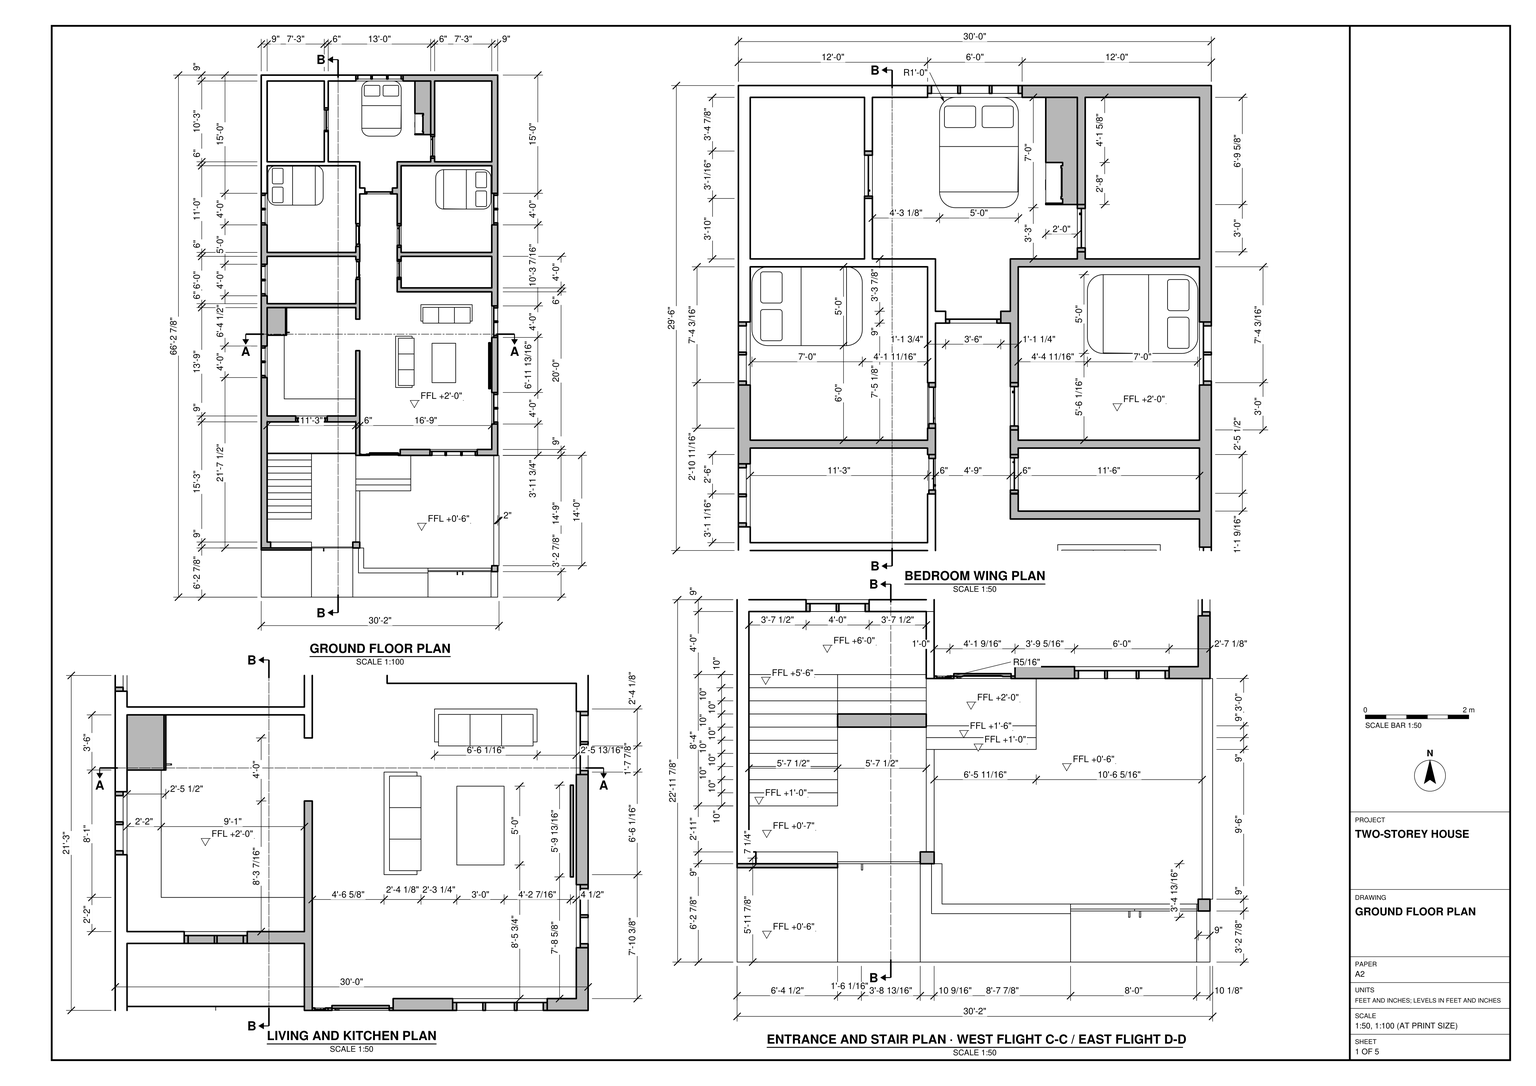
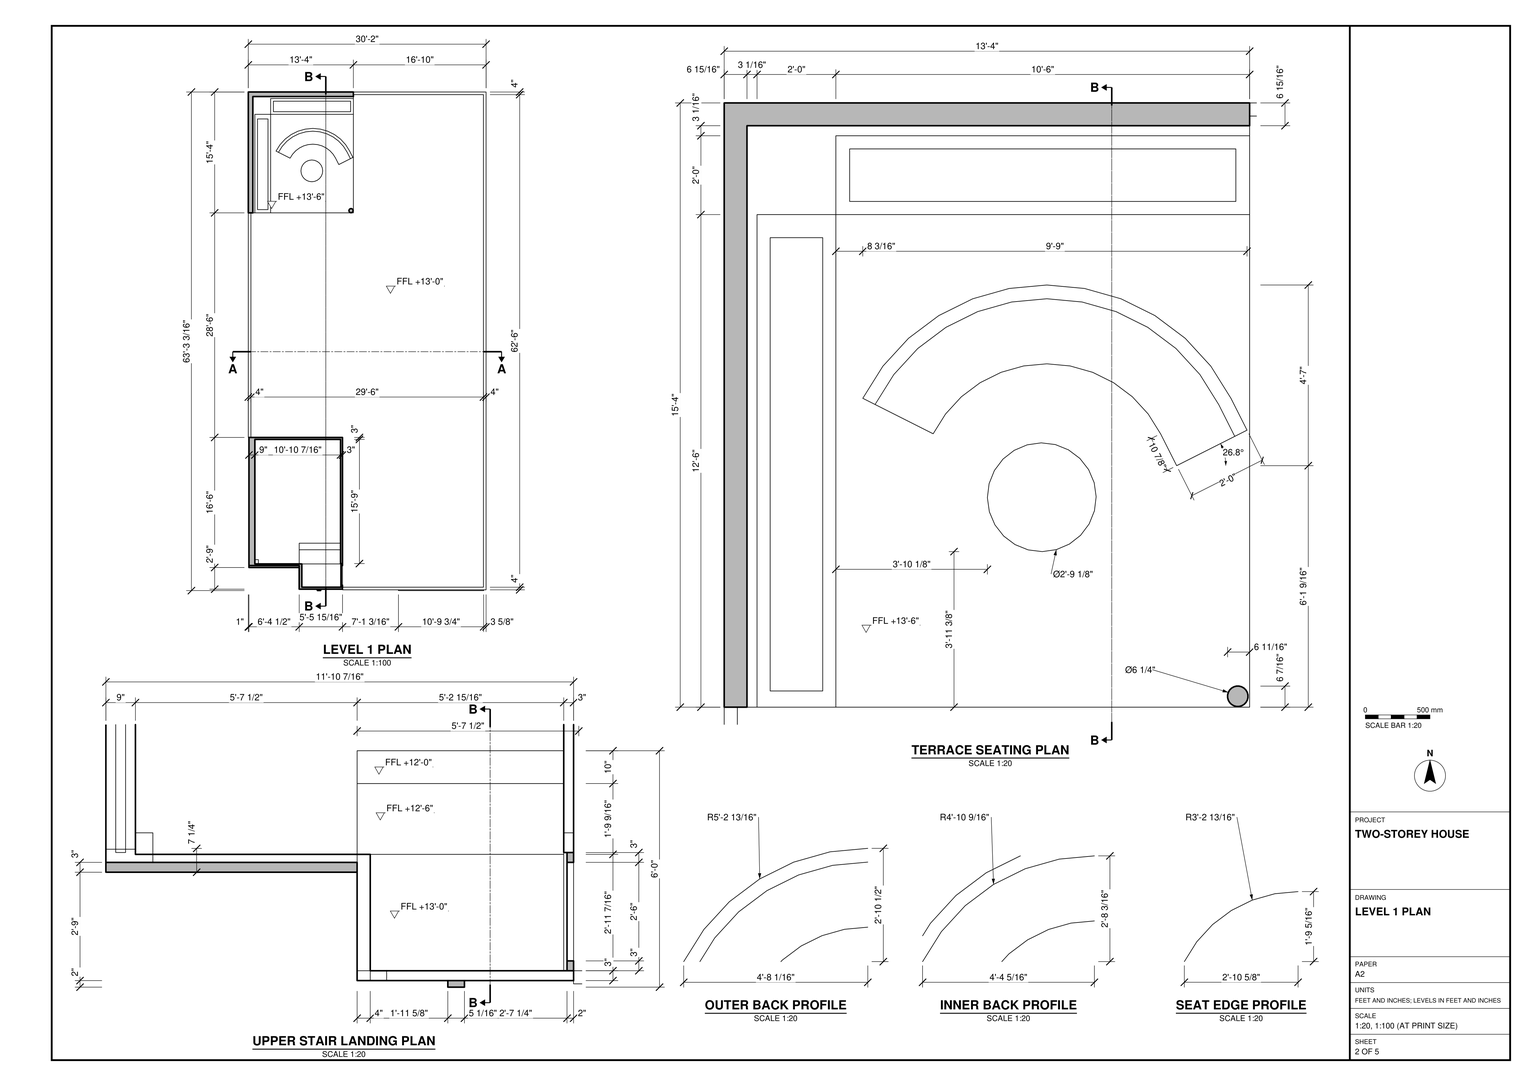
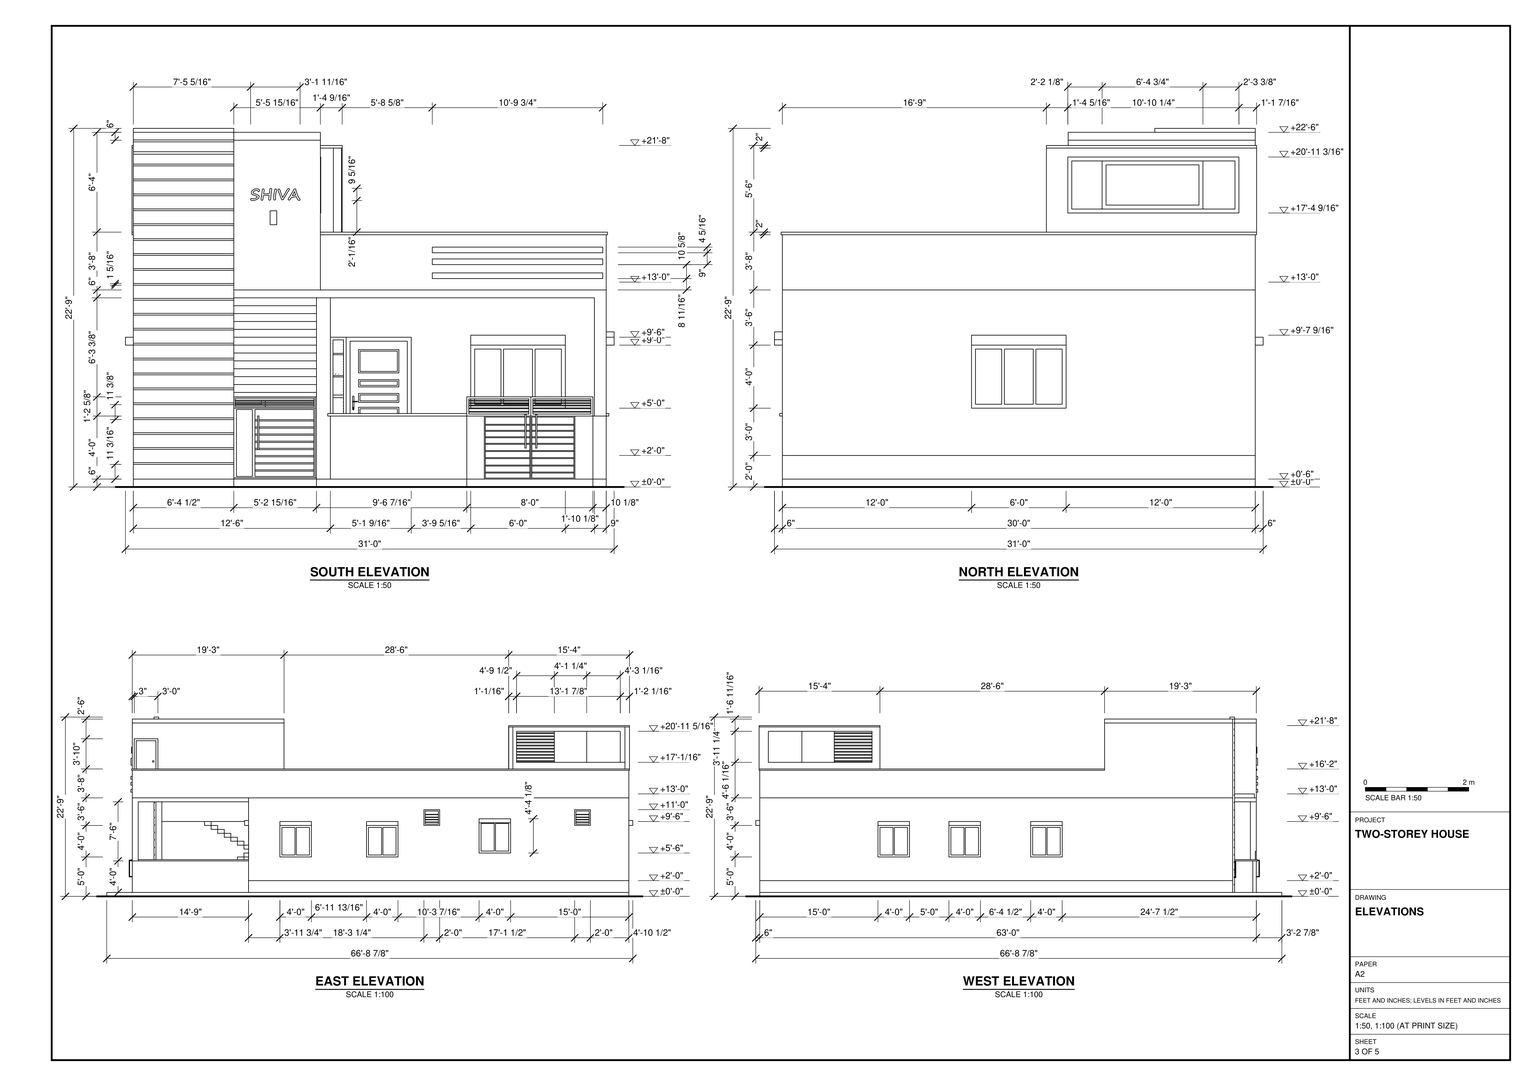
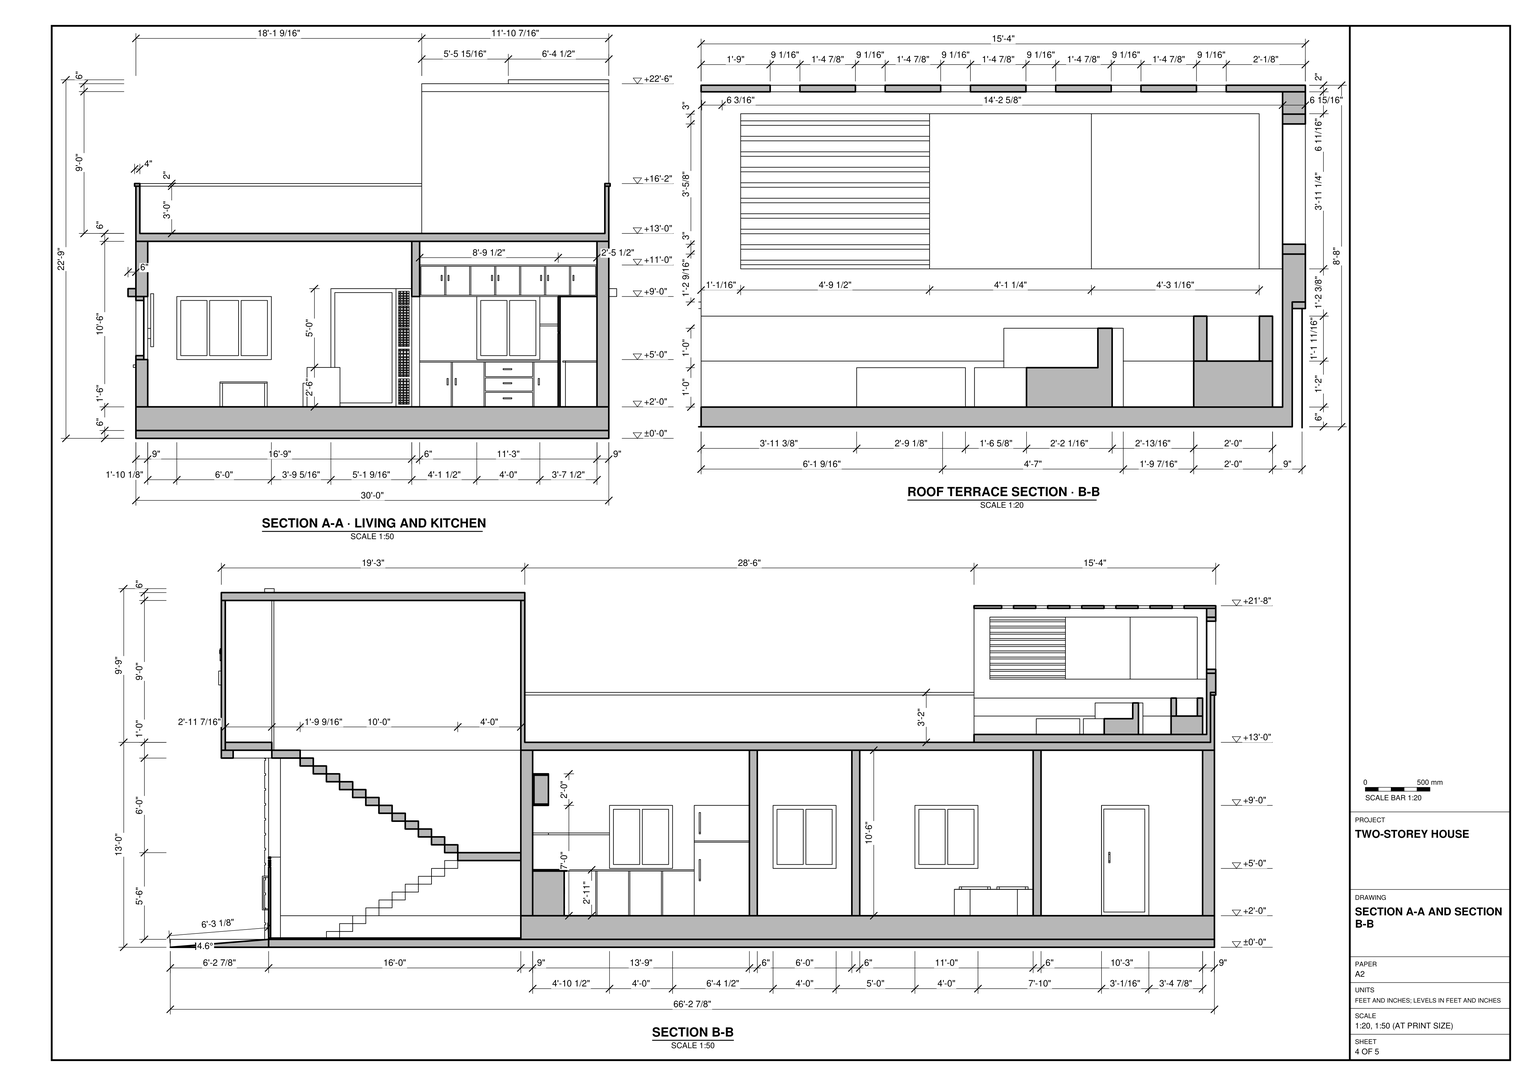
Build the house in SketchUp from task_files/diagram_01.pdf. Work in feet and inches. Set the overall width to 31'-0", the front-to-back length to 66'-8 7/8" and the height to 22'-9". Use ±0'-0" as the ground-floor datum and +13'-0" as the upper storey level. Distinguish these levels from the raised floor surfaces shown on the plans.

Start at the south entrance. Model the front gates, porch, entry steps and return stair, including its intermediate and upper landings. Place the living area and kitchen behind the porch, with a passage leading to the rear bedroom wing. Follow the drawn wall thicknesses, including the 9" exterior walls and 6" partitions where indicated. Form the door, window and vent openings to match the plans and elevations. Include the kitchen joinery, bedroom storage, beds, living room seating and rectangular table in their drawn positions.

Model the floor and roof slabs, terrace parapets and raised stair enclosure. At the opposite end of the terrace, reproduce the raised seating area with its curved seat and round table. Use the elevations to set out the horizontal bands on the entrance front and the openings along both sides. Decor and loose items may be any suitable library components.

Keep shell elements such as walls, slabs and roof, and each furniture or joinery piece, in separate groups or components. Use components for repeated parts. Save one SketchUp model as output_files/two_storey_house_with_a_furnished_roof_terrace.skp.

# SketchUp Ruby script. Lengths in inches.
U = 1.inch
M = Sketchup.active_model
def pt(a) = Geom::Point3d.new(a.map { |v| v * U })
def face(e, loops, mat)
  f = e.add_face(loops[0].map { |a| pt(a) })
  loops[1..].each { |l| e.add_face(l.map { |a| pt(a) }).erase! }
  f.material = f.back_material = mat if mat
  f
end
# faces: each face lists its corners as indices into pts; further lists are holes
def faces(e, pts, list, mat = nil) = list.each { |f| face(e, (f[0].is_a?(Array) ? f : [f]).map { |l| l.map { |i| pts[i] } }, mat) }
# xy, xz, yz: faces in a plane at the given z, y or x. An outline is a flat list of corners, or four numbers for a rectangle; further outlines are holes
def ring(l) = l.size == 4 ? [[l[0], l[1]], [l[2], l[1]], [l[2], l[3]], [l[0], l[3]]] : l.each_slice(2).to_a
def flat(e, list, mat, &to3) = list.each { |f| face(e, (f[0].is_a?(Array) ? f : [f]).map { |l| ring(l).map { |u, v| to3.(u, v) } }, mat) }
def xy(e, z, list, mat = nil) = flat(e, list, mat) { |x, y| [x, y, z] }
def xz(e, y, list, mat = nil) = flat(e, list, mat) { |x, z| [x, y, z] }
def yz(e, x, list, mat = nil) = flat(e, list, mat) { |y, z| [x, y, z] }
def lines(e, pts, list) = list.each { |a, b| e.add_line(pt(pts[a]), pt(pts[b])) }
# prism: a flat outline (further loops are holes) pulled along v
def prism(e, loops, v, mat = nil)
  f = face(e, loops, mat); d = Geom::Vector3d.new(v.map { |x| x * U })
  f.pushpull(f.normal.samedirection?(d) ? d.length : -d.length)
end
def box(e, o, s, mat = nil) = prism(e, [[o, [o[0] + s[0], o[1], o[2]], [o[0] + s[0], o[1] + s[1], o[2]], [o[0], o[1] + s[1], o[2]]]], [0, 0, s[2]], mat)
def at(x, y, z, deg = 0) = Geom::Transformation.translation(pt([x, y, z])) * Geom::Transformation.rotation(ORIGIN, Z_AXIS, deg.degrees)
def axes(o, x, y, z) = Geom::Transformation.new([*x, 0, *y, 0, *z, 0, *pt(o).to_a, 1])
def part(name) = M.definitions.add(name)
# library, detail: a bought-in or finely detailed component or shape, given as its bounding box
def library(name, o, s) = part(name).tap { |d| box(d.entities, o, s) }
def detail(e, o, s) = box(e.add_group.entities, o, s)
def put(e, d, t, mat = nil) = e.add_instance(d, t).tap { |i| i.material = mat if mat }
def group(e, t, mat = nil) = e.add_group.tap { |g| g.transformation = t; g.material = mat if mat }.entities
root = M.entities
M.materials.add("A01_Blush_Petal").color = [255, 204, 204]
M.materials.add("B01_Ivory_Dust").color = [255, 217, 206]
M.materials.add("Carpet_1_1K").color = [242, 174, 12]
M.materials.add("G01_Mint_Mist").color = [204, 255, 204]
M.materials.add("Glass_Basic_01").color = [161, 173, 186]
M.materials["Glass_Basic_01"].alpha = 0.25
M.materials.add("Glass_Mirror_01").color = [185, 185, 185]
M.materials.add("M00_Soft_Cloud").color = [255, 255, 255]
M.materials.add("M02_Ash_Whisper").color = [196, 196, 196]
M.materials.add("M04_Stone_Frost").color = [142, 142, 142]
M.materials.add("M05_Graphite_Haze").color = [114, 114, 114]
M.materials.add("M06_Steel_Smoke").color = [86, 86, 86]
M.materials.add("M07_Charcoal_Gleam").color = [58, 58, 58]
M.materials.add("M08_Obsidian_Black").color = [30, 30, 30]
M.materials.add("M09_Shadow_Night").color = [0, 0, 0]
M.materials.add("Marble_01_1K").color = [230, 221, 211]
M.materials.add("Marble_03_1K").color = [175, 182, 201]
M.materials.add("Marble_06_1K").color = [165, 150, 147]
M.materials.add("Marble_20_1K").color = [172, 173, 182]
M.materials.add("Metal_06_1K").color = [220, 236, 231]
M.materials.add("Metal_10_1K").color = [196, 175, 123]
M.materials.add("Plaster_02_1K").color = [157, 140, 119]
M.materials.add("Plaster_04_1K").color = [106, 98, 87]
M.materials.add("Plywood_01_1K").color = [125, 96, 64]
M.materials.add("Soil_04_1K").color = [152, 146, 88]
M.materials.add("Wood_Floor_01_1K").color = [146, 111, 76]
M.materials.add("Wood_Floor_12_1K").color = [92, 75, 65]
M.materials.add("Wood_Veneer_15_1K").color = [103, 69, 45]
c1 = library("SHIVA",[0.42,0,0],[37.67,9.31,1])
c2 = part("Group\#4")
xy(c2.entities,0,[[0,-6,72,0]],"M09_Shadow_Night")
xy(c2.entities,3,[[3,-6,23,0],[25,-6,47,0],[49,-6,69,0]],"M09_Shadow_Night")
xy(c2.entities,45,[[3,-6,23,0],[25,-6,47,0],[49,-6,69,0]],"M09_Shadow_Night")
xy(c2.entities,48,[[0,-6,72,0]],"M09_Shadow_Night")
xz(c2.entities,-6,[[[0,0,72,48],[25,3,47,45],[3,3,23,45],[49,3,69,45]]],"M09_Shadow_Night")
xz(c2.entities,0,[[3,3,23,45],[25,3,47,45],[49,3,69,45]],"Glass_Basic_01")
xz(c2.entities,0,[[[0,0,72,48],[25,3,47,45],[3,3,23,45],[49,3,69,45]]],"M09_Shadow_Night")
yz(c2.entities,0,[[-6,0,0,48]],"M09_Shadow_Night")
yz(c2.entities,3,[[-6,3,0,45]],"M09_Shadow_Night")
yz(c2.entities,23,[[-6,3,0,45]],"M09_Shadow_Night")
yz(c2.entities,25,[[-6,3,0,45]],"M09_Shadow_Night")
yz(c2.entities,47,[[-6,3,0,45]],"M09_Shadow_Night")
yz(c2.entities,49,[[-6,3,0,45]],"M09_Shadow_Night")
yz(c2.entities,69,[[-6,3,0,45]],"M09_Shadow_Night")
yz(c2.entities,72,[[-6,0,0,48]],"M09_Shadow_Night")
c3 = part("Group\#5")
box(c3.entities,[0,-6,0],[72,6,7.5625])
c4 = library("Group\#14",[0,0,0],[6,36,90])
c5 = library("Group\#11",[0,-3,0],[42,3,84])
c6 = library("Group\#15",[0,0,0],[5,30,84])
c7 = library("Group\#17",[0,0,0],[6,34.6875,90])
c8 = library("Group\#18",[0,-1.85,0],[61.58,3.7,90])
c9 = library("Group\#37",[-11.5625,0,0],[62.92,1.5,62.625])
c10 = part("Group\#39")
xy(c10.entities,0,[[0,-24.625,1.0625,-23.8125],[0,0,1.0625,1.0625]],"Metal_06_1K")
xy(c10.entities,4,[[0,-23.8125,1.0625,0]],"M07_Charcoal_Gleam")
xy(c10.entities,4.8125,[[0,-24.625,1.0625,1.0625]],"Metal_06_1K")
xz(c10.entities,-24.625,[[0,0,1.0625,4.8125]],"Metal_06_1K")
xz(c10.entities,-23.8125,[[0,0,1.0625,4]],"Metal_06_1K")
xz(c10.entities,0,[[0,0,1.0625,4]],"Metal_06_1K")
xz(c10.entities,1.0625,[[0,0,1.0625,4.8125]],"Metal_06_1K")
yz(c10.entities,0,[[-24.625,0,-24.625,4.8125,1.0625,4.8125,1.0625,0,0,0,0,4,-23.8125,4,-23.8125,0]],"Metal_06_1K")
yz(c10.entities,1.0625,[[-24.625,0,-23.8125,0,-23.8125,4,0,4,0,0,1.0625,0,1.0625,4.8125,-24.625,4.8125]],"Metal_06_1K")
c11 = part("Group\#6")
xy(c11.entities,0,[[0,0,6,48]],"M09_Shadow_Night")
xy(c11.entities,3,[[0,3,6,23],[0,25,6,45]],"M09_Shadow_Night")
xy(c11.entities,45.02,[[0,3,6,23],[0,25,6,45]],"M09_Shadow_Night")
xy(c11.entities,48.02,[[0,0,6,48]],"M09_Shadow_Night")
xz(c11.entities,0,[[0,0,6,48.02]],"M09_Shadow_Night")
xz(c11.entities,3,[[0,3,6,45.02]],"M09_Shadow_Night")
xz(c11.entities,23,[[0,3,6,45.02]],"M09_Shadow_Night")
xz(c11.entities,25,[[0,3,6,45.02]],"M09_Shadow_Night")
xz(c11.entities,45,[[0,3,6,45.02]],"M09_Shadow_Night")
xz(c11.entities,48,[[0,0,6,48.02]],"M09_Shadow_Night")
yz(c11.entities,0,[[3,3,23,45.02],[25,3,45,45.02]],"Glass_Basic_01")
yz(c11.entities,0,[[[0,0,48,48.02],[3,3,23,45.02],[25,3,45,45.02]]],"M09_Shadow_Night")
yz(c11.entities,6,[[[0,0,48,48.02],[3,3,23,45.02],[25,3,45,45.02]]],"M09_Shadow_Night")
c12 = part("Group\#30")
box(c12.entities,[0,0,0],[6,48,6])
c13 = library("Group\#8",[0,0,0],[3,24,24])
c14 = library("Group\#40",[0,0,0],[2,36,84])
c15 = part("Group\#33")
box(c15.entities,[0,0,0],[67.5,10,6])
c16 = part("Group\#35")
box(c16.entities,[0,0,0],[67.5,10,6])
c17 = library("Group\#38",[0,-3,0],[76.5,7.25,200.25])
c18 = library("Group\#46",[0,0,0],[78.07,28.13,30])
c19 = library("Group\#52",[0,0,0],[135,165,84])
c20 = library("Group\#56",[-91.5,0,0],[135,12.21,24])
c21 = library("Group\#63",[0,0,0],[84,60,22])
c22 = library("Group\#62",[0,0,0],[84,60,22])
c23 = library("Group\#64",[-4.125,0,0],[28.125,72,114.1875])
c24 = part("Group\#68")
box(c24.entities,[0,-2.1875,0],[129.75,2.1875,4.3125])
c25 = library("Group\#73",[-4,0,0],[160,184,104])
c26 = library("Group\#81",[0,-9.71,0],[117,55.02,24])
c27 = library("Group\#82",[0,0,0],[33.125,33.125,12])
box(root,[266.05,326.59,24],[2,2,18])
box(root,[300.05,326.59,24],[2,2,18])
box(root,[300.05,384.59,24],[2,2,18])
box(root,[266.05,384.59,24],[2,2,18])
xy(root,0,[[6,74.875,366,794.875]])
p = [[150,266.875,6],[15,266.875,6],[15,128.875,6],[150,118.875,6],[82.5,118.875,6],[82.5,128.875,6],
  [824.34,221.29,0],[824.34,221.52,0],[1107.31,455.52,0],[1106.83,455.82,0],[1591.35,295.77,0],[1591.35,295.2,0],
  [1562.52,295.77,0],[1562.52,295.2,0],[1113.81,793.06,0],[1111.77,793.06,0]]
lines(root,p,[[0,1],[2,1],[3,0],[4,5],[5,2],[6,7],[8,9],[10,11],[12,13],[14,15]])
put(root,c1,axes([94.88,38.875,218.06],[1,0,0],[0,0,1],[0,-1,0]))
g1 = group(root,at(6,74.875,0))
xy(g1,0,[[0,0,360,720]])
g2 = group(root,at(30.7,105.14,0))
xy(g2,0,[[-24.7,-105.14,-24.7,689.74,335.3,689.74,335.3,-105.14,325.17,-105.14,325.17,-66.26,229.17,-66.26,229.17,-105.14,114.72,-105.14,114.72,-30.26,51.8,-30.26,51.8,-105.14],[51.8,-105.14,114.72,-30.26],[229.17,-105.14,325.17,-66.26]])
xy(g2,6,[[-24.7,-105.14,51.8,-105.14,51.8,-30.26,114.72,-30.26,114.72,-105.14,229.17,-105.14,229.17,-66.26,325.17,-66.26,325.17,-105.14,335.3,-105.14,335.3,689.74,-24.7,689.74]],"Plaster_02_1K")
xz(g2,-105.14,[[-24.7,0,51.8,6],[114.72,0,229.17,6],[325.17,0,335.3,6]],"Plaster_02_1K")
xz(g2,-66.26,[[229.17,0,325.17,6]])
xz(g2,-30.26,[[51.8,0,114.72,6]])
xz(g2,689.74,[[-24.7,0,335.3,6]],"Plaster_02_1K")
yz(g2,-24.7,[[-105.14,0,689.74,6]],"Plaster_02_1K")
yz(g2,51.8,[[-105.14,0,-30.26,0,-30.26,6]])
yz(g2,51.8,[[-105.14,0,-30.26,6,-105.14,6]],"Plaster_02_1K")
yz(g2,114.72,[[-105.14,0,-30.26,6,-30.26,0]])
yz(g2,114.72,[[-105.14,0,-105.14,6,-30.26,6]],"Plaster_02_1K")
yz(g2,229.17,[[-105.14,0,-66.26,0,-66.26,6]])
yz(g2,229.17,[[-105.14,0,-66.26,6,-105.14,6]],"Plaster_02_1K")
yz(g2,325.17,[[-105.14,0,-66.26,6,-66.26,0]])
yz(g2,325.17,[[-105.14,0,-105.14,6,-66.26,6]],"Plaster_02_1K")
yz(g2,335.3,[[-105.14,0,689.74,6]],"Plaster_02_1K")
p = [[114.72,-105.14,0],[114.72,-30.26,6],[51.8,-30.26,6],[51.8,-105.14,0],[325.17,-105.14,0],[325.17,-66.26,6],
  [229.17,-66.26,6],[229.17,-105.14,0]]
faces(g2,p,[[0,1,2,3],[4,5,6,7]],"Plaster_02_1K")
g3 = group(root,at(6,518.875,6),"Marble_01_1K")
xy(g3,0,[[150,-480,253.87,-474.6875],[253.87,-480,349.87,-474.6875],[349.87,-480,349.87,-474.6875,354,-474.6875,354,-444,360,-444,360,-480],[150,-474.6875,156,-444],[0,-444,76.5,-444,76.5,-435,9,-435,9,-252,144,-252,144,-435,139.42,-435,139.42,-444,150,-444,150,-303,360,-303,360,276,0,276],
  [150,-357,227.6875,-303]])
xy(g3,1,[[76.5,-444,139.42,-444,139.42,-435,144,-435,144,-252,9,-252,9,-435,76.5,-435]],"Marble_01_1K")
xy(g3,1,[[156,-474.6875,156,-444,150,-444,150,-357,227.6875,-357,227.6875,-303,354,-303,354,-474.6875]],"Soil_04_1K")
xy(g3,6,[[144,-435,150,-357]])
xy(g3,6,[[144,-357,227.6875,-348]],"Marble_20_1K")
xy(g3,12,[[144,-348,227.6875,-339]],"Marble_20_1K")
xy(g3,18,[[0,-444,0,-184.5,9,-184.5,9,-243,52.5,-243,52.5,-252,9,-252,9,-435,14.3125,-435,14.3125,-444],[211.58,-303,304.87,-294],[304.87,-303,328.87,-298.5],[328.87,-303,328.87,-294,351,-294,351,-207.27,360,-207.27,360,-303],[304.87,-298.5,328.87,-294],
  [52.5,-252,100.5,-243],[100.5,-252,100.5,-243,144,-243,144,-143.57,150,-143.57,150,-252],[351,-207.27,360,-123.43],[0,-184.5,0,-12,9,-12,9,-72,144,-72,144,-34.93,150,-34.93,150,-95.57,144,-95.57,144,-78,9,-78,9,-184.5],[351,-123.43,351,-54,207,-54,207,-34.93,213,-34.93,213,-48,351,-48,351,-12,360,-12,360,-123.43],
  [0,-12,0,48,9,48,9,6,144,6,144,12.49,150,12.49,150,-4.93,144,-4.93,144,0,9,0,9,-12],[351,-12,351,0,213,0,213,-4.93,207,-4.93,207,13.8,213,13.8,213,6,351,6,351,48,360,48,360,-12],[144,12.49,150,15.11],[0,48,0,276,144,276,144,267,102,267,102,226.1,96,226.1,96,267,9,267,9,144,96,144,96,190.1,102,190.1,102,144,150,144,150,104.125,157.75,104.125,157.75,95.125,150,95.125,150,49.8,144,49.8,144,138,9,138,9,48],[351,48,355.5,96],
  [355.5,48,360,96],[207,49.8,213,138],[199.75,95.125,207,104.125],[351,96,351,138,207,138,207,144,258,144,258,149.4,264,149.4,264,144,351,144,351,193.5,360,193.5,360,96],[258,185.4,258,267,192,267,192,276,360,276,360,193.5,351,193.5,351,267,264,267,264,185.4],
  [144,267,168,276],[168,267,192,276]])
xy(g3,18,[[150,-303,211.58,-303,211.58,-294,351,-294,351,-54,207,-54,207,-34.93,213,-34.93,213,-48,351,-48,351,0,213,0,213,-4.93,207,-4.93,207,95.125,150,95.125,150,-95.57,144,-95.57,144,-78,9,-78,9,-243,144,-243,144,-143.57,150,-143.57]],"Marble_01_1K")
xy(g3,18,[[9,-72,144,-72,144,-34.93,150,-34.93,150,-4.93,144,-4.93,144,0,9,0]],"Marble_03_1K")
xy(g3,18,[[9,6,144,138],[213,6,351,6,351,138,213,138,213,49.8,207,49.8,207,13.8,213,13.8],[157.75,95.125,199.75,95.125,199.75,104.125,207,104.125,207,144,258,144,258,149.4,264,149.4,264,144,351,144,351,267,264,267,264,185.4,258,185.4,258,267,102,267,102,226.1,96,226.1,96,267,9,267,9,144,96,144,96,190.1,102,190.1,102,144,150,144,150,104.125,157.75,104.125]],"Marble_06_1K")
xy(g3,18,[[144,-339,227.6875,-303]],"Marble_20_1K")
xy(g3,48,[[150,-480,253.87,-474.6875],[349.87,-480,360,-480,360,-471,354,-471,354,-474.6875,349.87,-474.6875],[150,-474.6875,156,-444],[354,-471,360,-303]])
xy(g3,48,[[148,-482,253.87,-480],[148,-480,150,-474.6875],[148,-474.6875,150,-444],[360,-471,362,-303]],"M00_Soft_Cloud")
xy(g3,49.9375,[[148,-482,253.87,-482,253.87,-474.6875,156,-474.6875,156,-444,148,-444]],"M00_Soft_Cloud")
xy(g3,50,[[354,-471,362,-303]],"M00_Soft_Cloud")
xy(g3,53.98,[[351,-255.27,360,-207.27]])
xy(g3,54,[[256.87,-303,328.87,-294],[52.5,-252,100.5,-243],[0,-184.5,9,-136.5],[351,-123.43,360,-75.43],[0,-60,9,-12],
  [0,48,9,96],[144,267,216,276]])
xy(g3,60,[[351,48,360,96]])
xy(g3,62.625,[[14.3125,-444,76.5,-435]],"G01_Mint_Mist")
xy(g3,102,[[256.87,-303,328.87,-294],[351,-255.27,360,-207.27],[52.5,-252,100.5,-247.5],[52.5,-247.5,100.5,-243],[0,-184.5,9,-136.5],
  [144,-143.57,150,-95.57],[351,-123.43,360,-75.43],[0,-60,9,-12],[351,-36,360,-12],[144,-34.93,150,-4.93],
  [207,-34.93,213,-4.93],[0,48,9,96],[157.75,95.125,199.75,104.125],[96,190.1,102,226.1],[351,193.5,360,217.5],
  [144,267,216,276]])
xy(g3,108,[[144,-435,150,-303],[150,-303,211.58,-294],[207,13.8,213,49.8],[351,48,355.5,96],[355.5,48,360,96],
  [258,149.4,264,185.4]])
xy(g3,108,[[144,15.11,150,49.8]],"Wood_Floor_12_1K")
xy(g3,126,[[351,-36,360,-12],[351,193.5,360,217.5]])
xy(g3,144,[[[0,-444,14.3125,-444,14.3125,-435,9,-435,9,-252,144,-252,144,-435,139.42,-435,139.42,-444,150,-444,150,-303,360,-303,360,276,0,276],[150,-294,150,95.125,207,95.125,207,-54,351,-54,351,-294],[9,-243,144,-78],[150,104.125,150,144,102,144,102,267,258,267,258,144,207,144,207,104.125],[213,6,351,138],[9,6,144,138],[9,144,96,267],[264,144,351,267],[9,-72,144,0],[213,-48,351,0]]])
xz(g3,-482,[[148,48,253.87,49.9375]],"M00_Soft_Cloud")
xz(g3,-480,[[150,0,253.87,48],[349.87,0,360,48]])
xz(g3,-474.6875,[[150,0,156,48],[156,1,253.87,48],[349.87,1,354,48]])
xz(g3,-474.6875,[[156,48,253.87,49.9375]],"M00_Soft_Cloud")
xz(g3,-474.6875,[[156,0,253.87,1],[253.87,0,349.87,1],[349.87,0,354,1]],"Soil_04_1K")
xz(g3,-471,[[354,48,362,50]],"M00_Soft_Cloud")
xz(g3,-444,[[150,1,156,48],[148,48,150,49.9375],[150,48,156,49.9375]])
xz(g3,-444,[[139.42,0,150,0,150,48,148,48,148,49.9375,150,49.9375,150,144,139.42,144],[0,18,14.3125,144]],"B01_Ivory_Dust")
xz(g3,-444,[[14.3125,0,76.5,62.625]],"G01_Mint_Mist")
xz(g3,-444,[[0,0,14.3125,18]],"M06_Steel_Smoke")
xz(g3,-444,[[76.5,0,139.42,1]],"Marble_01_1K")
xz(g3,-444,[[150,0,156,1]],"Soil_04_1K")
xz(g3,-435,[[139.42,1,144,144],[144,6,150,108]],"B01_Ivory_Dust")
xz(g3,-435,[[9,1,9,18,14.3125,18,14.3125,62.625,76.5,62.625,76.5,1],[9,18,14.3125,144]],"G01_Mint_Mist")
xz(g3,-435,[[9,0,76.5,1],[139.42,0,144,1]],"Marble_01_1K")
xz(g3,-357,[[150,1,227.6875,6]],"Marble_20_1K")
xz(g3,-357,[[150,0,227.6875,1]],"Soil_04_1K")
xz(g3,-348,[[144,6,227.6875,12]],"Marble_20_1K")
xz(g3,-339,[[144,12,227.6875,18]],"Marble_20_1K")
xz(g3,-303,[[354,0,360,18],[144,18,150,108],[354,18,360,48],[354,48,360,50],[360,48,362,50]])
xz(g3,-303,[[[211.58,18,354,18,354,50,360,50,360,144,150,144,150,108,211.58,108],[256.87,54,256.87,109.5625,320.74,109.5625,320.74,102,328.87,102,328.87,54]]],"B01_Ivory_Dust")
xz(g3,-303,[[227.6875,1,354,18]],"M06_Steel_Smoke")
xz(g3,-303,[[227.6875,0,354,1]],"Soil_04_1K")
xz(g3,-294,[[[211.58,18,211.58,108,150,108,150,144,351,144,351,18],[256.87,54,328.87,102]]])
xz(g3,-255.27,[[351,53.98,360,102]])
xz(g3,-252,[[[9,18,144,144],[52.5,54,100.5,102]]],"B01_Ivory_Dust")
xz(g3,-252,[[9,1,52.5,18],[52.5,1,100.5,18],[100.5,1,144,18]],"M06_Steel_Smoke")
xz(g3,-252,[[9,0,52.5,1],[52.5,0,100.5,1],[100.5,0,144,1]],"Marble_01_1K")
xz(g3,-243,[[[9,18,144,144],[52.5,54,100.5,102]]])
xz(g3,-207.27,[[351,53.98,360,102]])
xz(g3,-184.5,[[0,54,9,102]])
xz(g3,-143.57,[[144,18,150,102]])
xz(g3,-136.5,[[0,54,9,102]])
xz(g3,-123.43,[[351,54,360,102]])
xz(g3,-95.57,[[144,18,150,102]])
xz(g3,-78,[[9,18,144,144]])
xz(g3,-75.43,[[351,54,360,102]])
xz(g3,-72,[[9,18,144,144]])
xz(g3,-60,[[0,54,9,102]])
xz(g3,-54,[[207,18,351,144]])
xz(g3,-48,[[213,18,351,144]])
xz(g3,-36,[[351,102,360,126]])
xz(g3,-34.93,[[144,18,150,102],[207,18,213,102]])
xz(g3,-12,[[0,54,9,102],[351,102,360,126]])
xz(g3,-4.93,[[144,18,150,102],[207,18,213,102]])
xz(g3,0,[[9,18,144,144],[213,18,351,144]])
xz(g3,6,[[9,18,144,144],[213,18,351,144]])
xz(g3,13.8,[[207,18,213,108]])
xz(g3,15.11,[[144,18,150,108]])
xz(g3,48,[[0,54,9,102],[351,60,355.5,108],[355.5,60,360,108]])
xz(g3,49.8,[[207,18,213,108]])
xz(g3,95.125,[[150,18,157.75,18,157.75,102,199.75,102,199.75,18,207,18,207,144,150,144]])
xz(g3,96,[[0,54,9,102],[351,60,355.5,108],[355.5,60,360,108]])
xz(g3,104.125,[[150,18,150,144,207,144,207,18,199.75,18,199.75,102,157.75,102,157.75,18]])
xz(g3,138,[[207,0,213,6],[207,6,213,12],[207,12,213,18],[9,18,144,144],[213,18,351,144]])
xz(g3,144,[[9,18,96,144],[102,18,150,144],[207,18,258,144],[264,18,351,144]])
xz(g3,149.4,[[258,18,264,108]])
xz(g3,185.4,[[258,18,264,108]])
xz(g3,190.1,[[96,18,102,102]])
xz(g3,193.5,[[351,102,360,126]])
xz(g3,217.5,[[351,102,360,126]])
xz(g3,226.1,[[96,18,102,102]])
xz(g3,267,[[9,18,96,144],[[102,18,258,144],[144,54,216,102]],[264,18,351,144]])
xz(g3,276,[[[0,18,360,144],[144,54,216,102]]],"B01_Ivory_Dust")
xz(g3,276,[[0,0,360,18]],"M06_Steel_Smoke")
yz(g3,0,[[[-444,18,276,144],[-184.5,54,-136.5,102],[-60,54,-12,102],[48,54,96,102]]],"B01_Ivory_Dust")
yz(g3,0,[[-444,0,276,18]],"M06_Steel_Smoke")
yz(g3,9,[[-243,18,-78,18,-78,144,-243,144,-243,81,-184.5,81,-184.5,102,-136.5,102,-136.5,54,-184.5,54,-184.5,79.6,-243,79.6],[[-72,18,0,144],[-60,54,-12,102]],[[6,18,138,144],[48,54,96,102]],[144,18,267,144]])
yz(g3,9,[[-435,18,-252,144]],"B01_Ivory_Dust")
yz(g3,9,[[-435,1,-252,18]],"M06_Steel_Smoke")
yz(g3,9,[[-435,0,-252,1]],"Marble_01_1K")
yz(g3,14.3125,[[-444,62.625,-435,144]],"B01_Ivory_Dust")
yz(g3,14.3125,[[-444,18,-435,62.625]],"M06_Steel_Smoke")
yz(g3,52.5,[[-252,54,-247.5,102],[-247.5,54,-243,102]])
yz(g3,76.5,[[-444,1,-435,62.625]],"G01_Mint_Mist")
yz(g3,76.5,[[-444,0,-435,1]],"Marble_01_1K")
yz(g3,96,[[144,18,144,144,267,144,267,18,226.1,18,226.1,102,190.1,102,190.1,18]])
yz(g3,100.5,[[-252,54,-247.5,102],[-247.5,54,-243,102]])
yz(g3,102,[[144,18,190.1,18,190.1,102,226.1,102,226.1,18,267,18,267,144,144,144]])
yz(g3,139.42,[[-444,1,-435,144]],"B01_Ivory_Dust")
yz(g3,139.42,[[-444,0,-435,1]],"Marble_01_1K")
yz(g3,144,[[-435,1,-357,6],[-243,18,-243,144,-78,144,-78,18,-95.57,18,-95.57,102,-143.57,102,-143.57,18],[-72,18,-72,144,0,144,0,18,-4.93,18,-4.93,102,-34.93,102,-34.93,18],[267,54,276,102]])
yz(g3,144,[[-300,0,-300.17,1,-300,1],[-300.17,1,-303,18,-303,108,-435,108,-435,144,-294,144,-294,1],[-294,1,-252,144]],"B01_Ivory_Dust")
yz(g3,144,[[-435,0,-357,1],[-357,0,-348,1],[-348,0,-339,1],[-339,0,-303,1],[-303,0,-300,0,-300.17,1,-303,1],
  [-300,0,-294,1],[-294,0,-252,1],[-357,1,-348,6],[-348,1,-339,12],[-339,1,-303,18],
  [-303,1,-303,18,-300.17,1]],"Marble_01_1K")
yz(g3,144,[[6,18,6,144,138,144,138,18,49.8,18,49.8,108,15.11,108,15.11,18]],"Wood_Floor_12_1K")
yz(g3,148,[[-482,48,-444,49.9375]],"M00_Soft_Cloud")
yz(g3,150,[[-480,0,-474.6875,48],[-474.6875,0,-444,48],[-435,1,-357,6],[-303,18,-294,108],[-294,18,-143.57,18,-143.57,102,-95.57,102,-95.57,18,-34.93,18,-34.93,102,-4.93,102,-4.93,18,15.11,18,15.11,108,49.8,108,49.8,18,95.125,18,95.125,144,-294,144],
  [104.125,18,144,144],[-435,108,-303,144]])
yz(g3,150,[[-444,1,-435,144]],"B01_Ivory_Dust")
yz(g3,150,[[-444,0,-435,1],[-435,0,-357,1]],"Soil_04_1K")
yz(g3,156,[[-474.6875,1,-444,48]])
yz(g3,156,[[-474.6875,48,-444,49.9375]],"M00_Soft_Cloud")
yz(g3,156,[[-474.6875,0,-444,1]],"Soil_04_1K")
yz(g3,157.75,[[95.125,18,104.125,102]])
yz(g3,199.75,[[95.125,18,104.125,102]])
yz(g3,207,[[-54,18,-54,144,95.125,144,95.125,18,49.8,18,49.8,108,13.8,108,13.8,18,-4.93,18,-4.93,102,-34.93,102,-34.93,18],[104.125,18,144,144]])
yz(g3,211.58,[[-303,18,-294,108]])
yz(g3,213,[[-48,18,-34.93,18,-34.93,102,-4.93,102,-4.93,18,0,18,0,144,-48,144],[6,18,13.8,18,13.8,108,49.8,108,49.8,18,138,18,138,144,6,144]])
yz(g3,216,[[267,54,276,102]])
yz(g3,227.6875,[[-357,1,-348,6],[-348,1,-339,12],[-339,1,-303,18]],"Marble_20_1K")
yz(g3,227.6875,[[-357,0,-348,1],[-348,0,-339,1],[-339,0,-303,1]],"Soil_04_1K")
yz(g3,253.87,[[-480,0,-474.6875,48],[-482,48,-474.6875,49.9375]])
yz(g3,256.87,[[-303,54,-294,102]])
yz(g3,258,[[144,18,144,144,267,144,267,18,185.4,18,185.4,108,149.4,108,149.4,18]])
yz(g3,264,[[144,18,149.4,18,149.4,108,185.4,108,185.4,18,267,18,267,144,144,144]])
yz(g3,328.87,[[-303,54,-294,102]])
yz(g3,349.87,[[-480,0,-474.6875,48]])
yz(g3,351,[[[-294,18,-54,144],[-255.27,53.98,-207.27,102],[-123.43,54,-75.43,102]],[[-48,18,0,144],[-36,102,-12,126]],[[6,18,138,144],[48,60,96,108]],[[144,18,267,144],[193.5,102,217.5,126]]])
yz(g3,354,[[-474.6875,1,-303,48]])
yz(g3,354,[[-471,48,-303,50]],"M00_Soft_Cloud")
yz(g3,354,[[-474.6875,0,-444,1]],"Soil_04_1K")
yz(g3,360,[[-480,0,-303,48]])
yz(g3,360,[[[-303,18,276,144],[-255.27,53.98,-207.27,102],[48,60,96,108],[-123.43,54,-75.43,102],[193.5,102,217.5,126],[-36,102,-12,126]]],"B01_Ivory_Dust")
yz(g3,360,[[-303,0,276,18]],"M06_Steel_Smoke")
yz(g3,362,[[-471,48,-303,50]],"M00_Soft_Cloud")
p = [[355.5,-12,18],[355.5,-12,102],[150,12.49,108],[144,12.49,108],[52.5,-247.5,18],[52.5,-247.5,54],
  [100.5,-247.5,18],[100.5,-247.5,54],[355.5,96,108],[355.5,96,144],[355.5,48,18],[355.5,48,60],
  [355.5,48,108],[355.5,48,144],[355.5,96,18],[355.5,96,60]]
lines(g3,p,[[0,1],[2,3],[4,5],[6,7],[8,9],[10,11],[12,13],[14,15]])
put(g3,c2,at(256.87,-297,54))
put(g3,c3,at(256.87,-303,102),"M02_Ash_Whisper")
put(g3,c2,at(144,276,54))
put(g3,c3,at(144,282,102),"M02_Ash_Whisper")
put(g3,c4,at(207,13.8,18))
put(g3,c5,at(157.75,98.125,18))
put(g3,c6,at(145,-34.93,18))
put(g3,c4,axes([207,-34.45,18],[1,0,0],[0,0.82,0],[0,0,0.93333]))
put(g3,c4,at(258,149.4,18))
put(g3,c7,axes([96,190.02,18],[1,0,0],[0,1.04,0],[0,0,0.93333]))
put(g3,c6,axes([145,15.11,18],[1,0,0],[0,1.15625,0],[0,0,1.07143]))
g4 = group(g3,at(52.5,-246,54))
xy(g4,0,[[0,-6,48,0]],"M08_Obsidian_Black")
xy(g4,3,[[3,-6,23,0],[25,-6,45,0]],"M08_Obsidian_Black")
xy(g4,45,[[3,-6,23,0],[25,-6,45,0]],"M08_Obsidian_Black")
xy(g4,48,[[0,-6,48,0]],"M08_Obsidian_Black")
xz(g4,-6,[[[0,0,48,48],[3,3,23,45],[25,3,45,45]]],"M08_Obsidian_Black")
xz(g4,0,[[3,3,23,45],[25,3,45,45]],"Glass_Basic_01")
xz(g4,0,[[[0,0,48,48],[3,3,23,45],[25,3,45,45]]],"M08_Obsidian_Black")
yz(g4,0,[[-6,0,0,48]],"M08_Obsidian_Black")
yz(g4,3,[[-6,3,0,45]],"M08_Obsidian_Black")
yz(g4,23,[[-6,3,0,45]],"M08_Obsidian_Black")
yz(g4,25,[[-6,3,0,45]],"M08_Obsidian_Black")
yz(g4,45,[[-6,3,0,45]],"M08_Obsidian_Black")
yz(g4,48,[[-6,0,0,48]],"M08_Obsidian_Black")
put(g3,c8,at(150,-301.15,18),"Plywood_01_1K")
put(g3,c9,at(88.0625,-444,0))
g5 = group(g3,at(253.87,-480,0))
xy(g5,0,[[0,0,48.75,1.5],[48.75,0,96,1.5]],"M07_Charcoal_Gleam")
xy(g5,49.52,[[1.52,0,47.23,1.5],[50.27,0,94.48,1.5]],"M07_Charcoal_Gleam")
xy(g5,50.9375,[[1.52,0,47.23,1.5],[50.27,0,94.48,1.5]],"M07_Charcoal_Gleam")
xy(g5,51.55,[[1.52,0,47.23,1.5],[50.27,0,94.48,1.5]],"M07_Charcoal_Gleam")
xy(g5,53.58,[[1.52,0,47.23,1.5],[50.27,0,94.48,1.5]],"M07_Charcoal_Gleam")
xy(g5,54.1875,[[1.52,0,47.23,1.5],[50.27,0,94.48,1.5]],"M07_Charcoal_Gleam")
xy(g5,55.7,[[1.52,0,47.23,1.5],[50.27,0,94.48,1.5]],"M07_Charcoal_Gleam")
xy(g5,56.3125,[[1.52,0,47.23,1.5],[50.27,0,94.48,1.5]],"M07_Charcoal_Gleam")
xy(g5,57.52,[[1.52,0,47.23,1.5],[50.27,0,94.48,1.5]],"M07_Charcoal_Gleam")
xy(g5,58.125,[[1.52,0,47.23,1.5],[50.27,0,94.48,1.5]],"M07_Charcoal_Gleam")
xy(g5,59.375,[[1.52,0,47.23,1.5],[50.27,0,94.48,1.5]],"M07_Charcoal_Gleam")
xy(g5,59.99,[[1.52,0,47.23,1.5],[50.27,0,94.48,1.5]],"M07_Charcoal_Gleam")
xy(g5,61.11,[[1.52,0,47.23,1.5],[50.27,0,94.48,1.5]],"M07_Charcoal_Gleam")
xy(g5,62.625,[[0,0,48.75,1.5],[48.75,0,96,1.5]],"Metal_06_1K")
xz(g5,0,[[0,0,13.32,48],[82.3,0,96,48]],"Carpet_1_1K")
xz(g5,0,[[[13.32,0,48.75,48],[14.11,0.78,47.97,47.22]],[[48.75,0,82.3,48],[49.54,0.78,81.52,47.22]],[14.11,4.61,47.97,5.35],[49.54,4.61,81.52,5.35],[14.11,9.92,47.97,10.67],
  [49.54,9.92,81.52,10.67],[14.11,15.61,47.97,16.36],[49.54,15.61,81.52,16.36],[14.11,20.99,47.97,21.73],[49.54,20.99,81.52,21.73],
  [14.11,26.49,47.97,27.23],[49.54,26.49,81.52,27.23],[14.11,31.49,47.97,32.23],[49.54,31.49,81.52,32.23],[14.11,36.36,47.97,37.11],
  [49.54,36.36,81.52,37.11],[14.11,40.99,47.97,41.73],[49.54,40.99,81.52,41.73],[[0,48,48.75,62.625],[1.52,49.52,47.23,61.11]],[[48.75,48,96,62.625],[50.27,49.52,94.48,61.11]]],"Metal_06_1K")
xz(g5,0,[[1.52,50.9375,47.23,51.55],[50.27,50.9375,94.48,51.55],[1.52,53.58,47.23,54.1875],[50.27,53.58,94.48,54.1875],[1.52,55.7,47.23,56.3125],
  [50.27,55.7,94.48,56.3125],[1.52,57.52,47.23,58.125],[50.27,57.52,94.48,58.125],[1.52,59.375,47.23,59.99],[50.27,59.375,94.48,59.99]],"Metal_10_1K")
xz(g5,0,[[14.11,0.78,47.97,4.61],[49.54,0.78,81.52,4.61],[14.11,5.35,47.97,9.92],[49.54,5.35,81.52,9.92],[14.11,10.67,47.97,15.61],
  [49.54,10.67,81.52,15.61],[14.11,16.36,47.97,20.99],[49.54,16.36,81.52,20.99],[14.11,21.73,47.97,26.49],[49.54,21.73,81.52,26.49],
  [14.11,27.23,47.97,31.49],[49.54,27.23,81.52,31.49],[14.11,32.23,47.97,36.36],[49.54,32.23,81.52,36.36],[14.11,37.11,47.97,40.99],
  [49.54,37.11,81.52,40.99],[14.11,41.73,47.97,47.22],[49.54,41.73,81.52,47.22]],"Plywood_01_1K")
xz(g5,1.5,[[[0,0,48.75,62.625],[1.52,51.55,47.23,53.58],[1.52,54.1875,47.23,55.7],[1.52,49.52,47.23,50.9375],[1.52,58.125,47.23,59.375],[1.52,56.3125,47.23,57.52],[1.52,59.99,47.23,61.11]],[[48.75,0,96,62.625],[50.27,51.55,94.48,53.58],[50.27,54.1875,94.48,55.7],[50.27,49.52,94.48,50.9375],[50.27,58.125,94.48,59.375],[50.27,56.3125,94.48,57.52],[50.27,59.99,94.48,61.11]]],"Metal_06_1K")
yz(g5,0,[[0,0,1.5,62.625]],"Metal_06_1K")
yz(g5,1.52,[[0,49.52,1.5,50.9375],[0,51.55,1.5,53.58],[0,54.1875,1.5,55.7],[0,56.3125,1.5,57.52],[0,58.125,1.5,59.375],
  [0,59.99,1.5,61.11]],"M07_Charcoal_Gleam")
yz(g5,47.23,[[0,49.52,1.5,50.9375],[0,51.55,1.5,53.58],[0,54.1875,1.5,55.7],[0,56.3125,1.5,57.52],[0,58.125,1.5,59.375],
  [0,59.99,1.5,61.11]],"M07_Charcoal_Gleam")
yz(g5,48.75,[[0,0,1.5,62.625]],"M07_Charcoal_Gleam")
yz(g5,50.27,[[0,49.52,1.5,50.9375],[0,51.55,1.5,53.58],[0,54.1875,1.5,55.7],[0,56.3125,1.5,57.52],[0,58.125,1.5,59.375],
  [0,59.99,1.5,61.11]],"M07_Charcoal_Gleam")
yz(g5,94.48,[[0,49.52,1.5,50.9375],[0,51.55,1.5,53.58],[0,54.1875,1.5,55.7],[0,56.3125,1.5,57.52],[0,58.125,1.5,59.375],
  [0,59.99,1.5,61.11]],"M07_Charcoal_Gleam")
yz(g5,96,[[0,0,1.5,62.625]],"Metal_06_1K")
put(g5,c10,axes([44.16,0,48.22],[1,0,0],[0,0,1],[0,-1,0]))
put(g5,c10,axes([52.35,0,48.22],[1,0,0],[0,0,1],[0,-1,0]))
put(g5,c10,axes([-159.29,36,47.05],[1,0,0],[0,0,1],[0,-1,0]))
g6 = group(g3,at(9,-243,79.6),"Plywood_01_1K")
prism(g6,[[[0,0,0],[0,58.5,0],[12,58.5,0],[12,12,0],[43.5,12,0],[43.5,0,0]]],[0,0,1.4])
put(root,c11,at(360,263.61,59.98))
put(root,c12,at(366,263.61,108),"M02_Ash_Whisper")
put(root,c11,at(360,395.44,59.98))
put(root,c11,at(360,566.875,66))
put(root,c11,at(6,566.875,60))
put(root,c11,at(6,458.875,60))
put(root,c11,at(6,334.375,60))
put(root,c13,at(363,712.375,108))
put(root,c13,at(363,482.875,108))
put(root,c12,at(366,395.44,108),"M02_Ash_Whisper")
put(root,c12,at(366,566.875,112.11),"M02_Ash_Whisper")
g7 = group(root,at(0,566.875,108),"M02_Ash_Whisper")
box(g7,[0,0,0],[6,48,6])
put(root,c12,at(0,458.875,108),"M02_Ash_Whisper")
put(root,c12,at(0,334.375,108),"M02_Ash_Whisper")
g8 = group(root,at(6,215.875,150))
xy(g8,0,[[80.5,-177,80.5,-174,139.42,-174,139.42,51,9,51,9,-137,0,-137,0,579,360,579,360,-168,204,-168,204,-177],[76.5,-177,80.5,-174],[0,-141,0,-137,9,-137,9,-138.5625,76.5,-138.5625,76.5,-141]])
xy(g8,6,[[76.5,-174,80.5,-138.5625],[139.42,-174,142.42,-138]])
xy(g8,6,[[142.42,-174,357,-174,357,576,3,576,3,54,142.42,54]],"B01_Ivory_Dust")
xy(g8,42,[[142.42,-178,361,-177],[142.42,-177,360,-174],[360,-177,361,-174],[357,-174,357,576,3,576,3,54,0,54,0,579,360,579,360,-174],[360,-174,361,580],
  [-1,54,0,579],[-1,579,360,580]])
xy(g8,44,[[142.42,-178,361,-178,361,580,-1,580,-1,54,3,54,3,576,357,576,357,-174,142.42,-174]])
xy(g8,90,[[139.42,-174,142.42,-138]])
xy(g8,114,[[[76.5,-177,142.42,-177,142.42,54,0,54,0,-141,76.5,-141],[80.5,-174,80.5,-138.5625,9,-138.5625,9,51,139.42,51,139.42,-174]]])
xz(g8,-178,[[142.42,42,361,44]])
xz(g8,-177,[[142.42,0,360,42]],"B01_Ivory_Dust")
xz(g8,-177,[[76.5,0,142.42,114]],"Plaster_04_1K")
xz(g8,-174,[[76.5,0,80.5,6],[80.5,0,139.42,6],[80.5,6,139.42,114],[139.42,6,142.42,90],[142.42,6,357,42],
  [142.42,42,357,44]])
xz(g8,-141,[[0,0,76.5,114]])
xz(g8,-138.5625,[[9,0,76.5,114],[76.5,6,80.5,114]])
xz(g8,-138,[[139.42,6,142.42,90]])
xz(g8,51,[[9,0,139.42,114]],"Plaster_02_1K")
xz(g8,54,[[-1,42,0,44],[0,42,3,44]])
xz(g8,54,[[3,6,3,44,0,44,0,114,142.42,114,142.42,6]],"B01_Ivory_Dust")
xz(g8,576,[[3,42,357,44]])
xz(g8,576,[[3,6,357,42]],"B01_Ivory_Dust")
xz(g8,579,[[0,0,360,42]],"B01_Ivory_Dust")
xz(g8,580,[[-1,42,361,44]])
yz(g8,-1,[[54,42,580,44]])
yz(g8,0,[[-141,0,-141,114,54,114,54,42,579,42,579,0]],"B01_Ivory_Dust")
yz(g8,3,[[54,42,576,44]])
yz(g8,3,[[54,6,576,42]],"B01_Ivory_Dust")
yz(g8,9,[[-138.5625,0,-137,114],[-137,0,51,114]])
yz(g8,76.5,[[-141,0,-138.5625,6]])
yz(g8,76.5,[[-177,0,-177,114,-141,114,-141,6,-174,6,-174,0]],"Plaster_04_1K")
yz(g8,80.5,[[-174,6,-138.5625,114]])
yz(g8,139.42,[[-174,0,-174,6,-138,6,-138,90,-174,90,-174,114,51,114,51,0]])
yz(g8,142.42,[[-178,42,-177,44],[-177,42,-174,44]])
yz(g8,142.42,[[-138,6,54,6,54,114,-177,114,-177,44,-174,44,-174,90,-138,90]],"B01_Ivory_Dust")
yz(g8,357,[[-174,6,576,42],[-174,42,576,44]])
yz(g8,360,[[-177,0,579,42]],"B01_Ivory_Dust")
yz(g8,361,[[-178,42,580,44]])
p = [[3,-138,6],[6,-138,6],[6,54,6],[3,54,6]]
lines(g8,p,[[0,1],[1,2],[3,0]])
put(g8,c14,at(140.42,-174,6))
g9 = group(g8,at(204,-177,0),"Plaster_02_1K")
xy(g9,-96,[[147,0,156,9]],"M05_Graphite_Haze")
xy(g9,-6,[[-118.5,0,147,9]],"M04_Stone_Frost")
xy(g9,-6,[[-127.5,0,-118.5,38.4375],[147,9,156,177]],"M05_Graphite_Haze")
xy(g9,0,[[-127.5,0,-118.5,38.4375],[-118.5,0,147,9],[147,0,156,177]],"M04_Stone_Frost")
xz(g9,0,[[147,-96,156,-96,156,0,-127.5,0,-127.5,-6,147,-6]],"M04_Stone_Frost")
xz(g9,9,[[-118.5,-6,147,0]],"M04_Stone_Frost")
xz(g9,9,[[147,-96,156,-6]],"M05_Graphite_Haze")
xz(g9,38.4375,[[-127.5,-6,-118.5,0]],"M04_Stone_Frost")
xz(g9,177,[[147,-6,156,0]],"M04_Stone_Frost")
yz(g9,-127.5,[[0,-6,38.4375,0]],"M05_Graphite_Haze")
yz(g9,-118.5,[[9,-6,38.4375,0]],"M04_Stone_Frost")
yz(g9,147,[[0,-96,9,-6],[9,-6,177,0]],"M05_Graphite_Haze")
yz(g9,156,[[0,-96,9,-96,9,-6,177,-6,177,0,0,0]],"M05_Graphite_Haze")
put(root,c15,at(15,118.875,6),"Plywood_01_1K")
put(root,c15,at(15,128.875,12),"Plywood_01_1K")
put(root,c15,at(15,138.875,18),"Plywood_01_1K")
put(root,c15,at(15,148.875,24),"Plywood_01_1K")
put(root,c15,at(15,158.875,30),"Plywood_01_1K")
put(root,c15,at(15,168.875,36),"Plywood_01_1K")
put(root,c15,at(15,178.875,42),"Plywood_01_1K")
put(root,c15,at(15,188.875,48),"Plywood_01_1K")
put(root,c15,at(15,198.875,54),"Plywood_01_1K")
put(root,c16,at(15,208.875,60),"Plywood_01_1K")
g10 = group(root,at(15,218.875,66),"Plywood_01_1K")
box(g10,[0,0,0],[135,48,6])
put(root,c16,at(82.5,208.875,72),"Plywood_01_1K")
put(root,c16,at(82.5,198.875,78),"Plywood_01_1K")
put(root,c16,at(82.5,188.875,84),"Plywood_01_1K")
put(root,c16,at(82.5,178.875,90),"Plywood_01_1K")
put(root,c16,at(82.5,168.875,96),"Plywood_01_1K")
put(root,c16,at(82.5,158.875,102),"Plywood_01_1K")
put(root,c16,at(82.5,148.875,108),"Plywood_01_1K")
put(root,c16,at(82.5,138.875,114),"Plywood_01_1K")
put(root,c16,at(82.5,128.875,120),"Plywood_01_1K")
put(root,c16,at(82.5,118.875,126),"Plywood_01_1K")
put(root,c16,at(82.5,108.875,132),"Plywood_01_1K")
put(root,c16,at(82.5,98.875,138),"Plywood_01_1K")
g11 = group(root,at(82.5,88.875,144),"Plywood_01_1K")
box(g11,[0,-11.5625,0],[62.92,21.5625,6])
g12 = group(root,at(82.5,67.3125,150),"Plywood_01_1K")
xy(g12,0,[[0,-25.4375,62.92,10]])
xy(g12,6,[[0,-25.4375,62.92,10]])
xz(g12,-25.4375,[[0,0,62.92,6]])
xz(g12,10,[[0,0,62.92,6]])
yz(g12,0,[[-25.4375,0,10,6]],"Plaster_04_1K")
yz(g12,62.92,[[-25.4375,0,10,6]])
put(root,c17,axes([6,74.875,6],[1,0,0],[0,1,0],[0,0,1.33333]),"Wood_Veneer_15_1K")
g13 = group(root,at(6,38.875,264))
prism(g13,[[[0,231,0],[142.42,231,0],[142.42,0,0],[76.5,0,0],[76.5,36,0],[0,36,0]]],[0,0,6])
put(root,c18,at(249.08,417.21,24),"A01_Blush_Petal")
put(root,c18,at(238.78,319.24,24,90),"A01_Blush_Petal")
g14 = group(root,at(357,344.33,76.03))
box(g14,[-2.25,0,0],[2.25,21.6875,7.6875],"M09_Shadow_Night")
g15 = group(root,at(354.75,344.33,76.03))
xy(g15,-6.25,[[-2.25,-26.8125,0,43]],"M09_Shadow_Night")
xy(g15,34.125,[[-2.25,-26.8125,0,43]],"M09_Shadow_Night")
xz(g15,-26.8125,[[-2.25,-6.25,0,34.125]],"M09_Shadow_Night")
xz(g15,43,[[-2.25,-6.25,0,34.125]],"M09_Shadow_Night")
yz(g15,-2.25,[[-26.1,-5.53,42.28,33.41]],"Glass_Mirror_01")
yz(g15,-2.25,[[[-26.8125,-6.25,43,34.125],[-26.1,-5.53,42.28,33.41]]],"M09_Shadow_Night")
yz(g15,0,[[-26.8125,-6.25,43,34.125]],"M09_Shadow_Night")
g16 = group(root,at(266.05,326.59,24))
xy(g16,0,[[0,0,2,2],[34,0,36,2],[0,58,2,60],[34,58,36,60]])
g17 = group(root,at(266.05,326.59,42))
box(g17,[0,0,0],[36,60,1],"Glass_Basic_01")
put(root,c19,at(15,275.875,24))
put(root,c20,at(106.5,275.875,108),"B01_Ivory_Dust")
put(root,c21,at(16.3,596.875,24))
put(root,c21,at(355.68,650.92,24,-180))
put(root,c22,at(159.13,785.875,24,-90))
put(root,c23,axes([240,704.28,24],[1,0,0],[0,1.13333,0],[0,0,1]))
put(root,c24,at(233.6,38.875,178.3))
put(root,c24,at(233.6,38.875,169.3))
put(root,c24,at(233.6,38.875,158.68))
g18 = group(root,at(109.1875,38.875,195.41))
box(g18,[0.9375,-2,4.25],[5.0625,2,10.625],"M08_Obsidian_Black")
put(root,c25,at(9,611.875,156))
put(root,c26,at(47.2,695.12,162),"Marble_06_1K")
put(root,c27,at(85.14,659.24,162),"Wood_Floor_01_1K")
